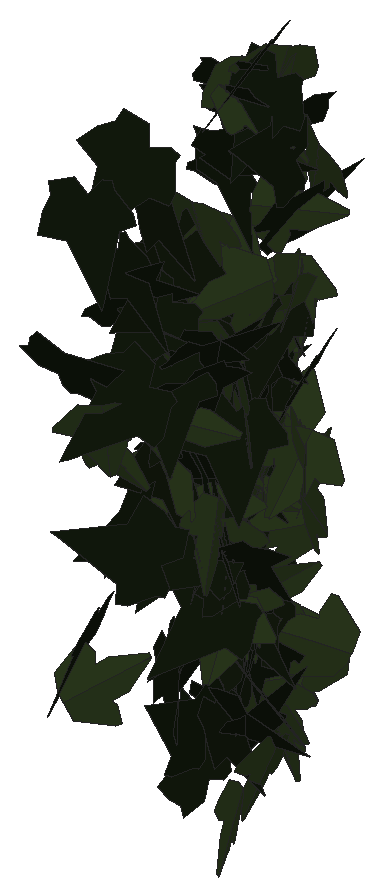
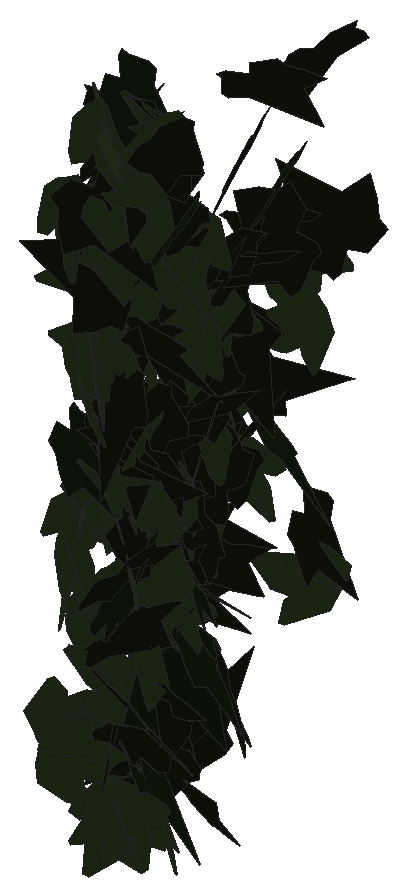
# SketchUp Ruby script. Lengths in inches.
U = 1.inch
M = Sketchup.active_model
def pt(a) = Geom::Point3d.new(a.map { |v| v * U })
def face(e, loops, mat)
  f = e.add_face(loops[0].map { |a| pt(a) })
  loops[1..].each { |l| e.add_face(l.map { |a| pt(a) }).erase! }
  f.material = f.back_material = mat if mat
  f
end
# faces: each face lists its corners as indices into pts; further lists are holes
def faces(e, pts, list, mat = nil) = list.each { |f| face(e, (f[0].is_a?(Array) ? f : [f]).map { |l| l.map { |i| pts[i] } }, mat) }
# xy, xz, yz: faces in a plane at the given z, y or x. An outline is a flat list of corners, or four numbers for a rectangle; further outlines are holes
def ring(l) = l.size == 4 ? [[l[0], l[1]], [l[2], l[1]], [l[2], l[3]], [l[0], l[3]]] : l.each_slice(2).to_a
def flat(e, list, mat, &to3) = list.each { |f| face(e, (f[0].is_a?(Array) ? f : [f]).map { |l| ring(l).map { |u, v| to3.(u, v) } }, mat) }
def xy(e, z, list, mat = nil) = flat(e, list, mat) { |x, y| [x, y, z] }
def xz(e, y, list, mat = nil) = flat(e, list, mat) { |x, z| [x, y, z] }
def yz(e, x, list, mat = nil) = flat(e, list, mat) { |y, z| [x, y, z] }
def lines(e, pts, list) = list.each { |a, b| e.add_line(pt(pts[a]), pt(pts[b])) }
# prism: a flat outline (further loops are holes) pulled along v
def prism(e, loops, v, mat = nil)
  f = face(e, loops, mat); d = Geom::Vector3d.new(v.map { |x| x * U })
  f.pushpull(f.normal.samedirection?(d) ? d.length : -d.length)
end
def box(e, o, s, mat = nil) = prism(e, [[o, [o[0] + s[0], o[1], o[2]], [o[0] + s[0], o[1] + s[1], o[2]], [o[0], o[1] + s[1], o[2]]]], [0, 0, s[2]], mat)
def at(x, y, z, deg = 0) = Geom::Transformation.translation(pt([x, y, z])) * Geom::Transformation.rotation(ORIGIN, Z_AXIS, deg.degrees)
def axes(o, x, y, z) = Geom::Transformation.new([*x, 0, *y, 0, *z, 0, *pt(o).to_a, 1])
def part(name) = M.definitions.add(name)
# library, detail: a bought-in or finely detailed component or shape, given as its bounding box
def library(name, o, s) = part(name).tap { |d| box(d.entities, o, s) }
def detail(e, o, s) = box(e.add_group.entities, o, s)
def put(e, d, t, mat = nil) = e.add_instance(d, t).tap { |i| i.material = mat if mat }
def group(e, t, mat = nil) = e.add_group.tap { |g| g.transformation = t; g.material = mat if mat }.entities
root = M.entities
M.materials.add("efeu1").color = [18, 25, 13]
M.materials.add("efeu2").color = [43, 57, 29]
c1 = part("ivyleaf_9")
p = [[1.54,2.16,1.25],[1.36,2.04,1.19],[-0.21,0.99,0.68],[-0.71,1.11,0.82],[-0.85,0.86,0.67],[-0.8,0.17,0.21],
  [-0.9,-0.01,0.1],[-0.67,-0.16,-0.02],[-0.08,-0.08,-0.05],[-0.03,-0.6,-0.4],[0.65,-0.88,-0.66],[0.83,-0.6,-0.49],
  [1.29,-0.42,-0.43],[1.8125,-0.07,-0.26],[1.21,0.44,0.15]]
faces(c1.entities,p,[[0,1,2,3,4,5,6,7,8,9,10,11,12,13,14]],"efeu1")
c2 = part("ivyleaf_10")
p = [[0,0.5,-0.03],[-0.0625,2.02,-0.43],[-0.19,2.01,-0.46],[-0.54,1.05,-0.29],[-0.52,0.625,-0.18],[-0.83,0.76,-0.28],
  [-1.16,0.64,-0.33],[-1.15,0.33,-0.24],[-0.77,-0.39,0.02],[-0.3,-0.51,0.16],[0.04,-0.48,0.23],[-0.02,2.01,-0.4375],
  [-0.06,2.01,-0.43],[0.04,-0.49,0.23],[0.67,-0.49,0.14],[1.38,0.36,-0.2],[1.375,0.51,-0.24],[0.81,0.65,-0.19],
  [0.62,0.59,-0.15],[0.6,1.09,-0.28],[0.5,1.23,-0.31]]
faces(c2.entities,p,[[0,1,2,3,4,5,6,7,8,9,10],[11,12,0,13,14,15,16,17,18,19,20]],"efeu2")
put(root,c1,axes([52.49,219.07,230.18],[0.03355,-0.19875,0.45757],[0.42754,-0.22487,-0.12902],[0.25707,0.39992,0.15486]))
put(root,c2,axes([53.3,218.97,229.84],[-0.39077,-0.31074,-0.02717],[0.0214,0.01674,-0.49926],[0.31119,-0.39136,0.00022]))
put(root,c1,axes([53.72,219.3,230.26],[-0.45004,-0.19221,0.10255],[-0.09066,-0.04877,-0.48929],[0.19809,-0.459,0.00905]))
put(root,c1,axes([54.02,219.17,227.8],[-0.2114,0.01977,0.45268],[-0.45185,0.02806,-0.21224],[-0.03379,-0.49882,0.006]))
put(root,c1,axes([52.84,219.21,232.84],[0.00085,-0.48604,-0.11732],[0.00176,0.11732,-0.48604],[0.5,0.00041,0.00191]))
put(root,c1,axes([52.77,219.44,226.41],[-0.27604,0.24164,-0.33972],[0.2451,-0.23552,-0.36668],[-0.33723,-0.36897,0.01157]))
put(root,c2,axes([52.78,219.42,229.24],[-0.31286,0.0658,-0.38444],[0.37768,-0.07193,-0.31967],[-0.09737,-0.4904,-0.0047]))
put(root,c2,axes([52.71,219.21,225.41],[0.17923,0.11616,-0.45209],[0.38711,0.2336,0.21349],[0.26082,-0.42654,-0.00619]))
put(root,c1,axes([53.09,219.83,227.77],[-0.36743,0.3333,0.06248],[-0.04862,0.03939,-0.49607],[-0.3356,-0.37062,0.00346]))
put(root,c1,axes([52.82,220.43,233.02],[-0.41171,-0.28303,0.01984],[-0.01039,-0.01989,-0.4995],[0.28353,-0.4117,0.0105]))
put(root,c1,axes([52.59,220.2,231.49],[0.30591,-0.37984,-0.11018],[-0.06702,0.08749,-0.4877],[0.38978,0.31315,0.00262]))
put(root,c1,axes([53.1875,220.51,229.81],[-0.26806,-0.30832,-0.28824],[0.31945,0.07496,-0.37727],[0.27585,-0.38642,0.1568]))
put(root,c1,axes([52.45,220.15,230.8125],[0.28224,0.27787,0.30517],[0.2129,0.2187,-0.39603],[-0.35357,0.3535,0.00513]))
put(root,c1,axes([52.83,220.91,230.51],[-0.32883,-0.35018,0.13873],[-0.03254,-0.15706,-0.47357],[0.37525,-0.32047,0.0805]))
put(root,c1,axes([52.66,221.16,230.56],[-0.08705,-0.25552,0.42087],[-0.14402,-0.39549,-0.26989],[0.47083,-0.16821,-0.00474]))
put(root,c1,axes([53.45,220.52,229.71],[0.17913,0.46548,-0.03522],[-0.01706,-0.03117,-0.49874],[-0.4665,0.17988,0.00472]))
put(root,c1,axes([52.68,221.19,227.96],[0.20703,-0.32676,-0.31681],[0.16838,-0.26836,0.38682],[-0.42283,-0.26686,-0.00108]))
put(root,c1,axes([52.67,220.71,232.24],[0.30016,-0.29801,-0.26663],[-0.20004,0.17676,-0.42277],[0.34624,0.36048,-0.01311]))
put(root,c1,axes([52.84,220.81,229.63],[-0.10996,0.41296,-0.25955],[0.08139,-0.2468,-0.42716],[-0.48092,-0.13619,-0.01294]))
put(root,c2,axes([52.76,220.88,227.96],[0.46781,0.01762,-0.17561],[-0.17545,-0.00761,-0.46814],[-0.01917,0.49963,-0.00094]))
put(root,c2,axes([52.88,220.75,228.93],[-0.08972,-0.1035,-0.48087],[0.465,0.14154,-0.11723],[0.16039,-0.46825,0.07085]))
put(root,c2,axes([52.83,220.77,228.74],[-0.28235,0.34296,0.22947],[-0.20138,0.12817,-0.43934],[-0.36018,-0.34051,0.06575]))
put(root,c1,axes([53.14,220.8,230.125],[0.39895,0.2774,-0.11783],[-0.10096,-0.06117,-0.48586],[-0.28398,0.41147,0.00721]))
put(root,c1,axes([53.07,221.33,223.92],[0.0538,0.0666,0.49262],[-0.30402,-0.38762,0.0856],[0.39329,-0.30874,-0.00121]))
put(root,c2,axes([53.27,221.29,227.3],[-0.0076,-0.39344,0.30846],[0.25408,-0.26872,-0.3365],[0.43056,0.15163,0.20401]))
put(root,c1,axes([53.22,220.84,229.74],[0.22782,0.41878,-0.15074],[0.07738,0.12949,0.4767],[0.4383,-0.24053,-0.0058]))
put(root,c1,axes([53.31,221.375,226.94],[-0.37477,-0.22935,0.23863],[-0.19792,-0.13363,-0.43928],[0.26527,-0.42372,0.00937]))
put(root,c2,axes([53,221.125,229.96],[-0.29644,-0.40088,-0.03766],[0.02235,0.03031,-0.49858],[0.40203,-0.29728,-0.00005]))
put(root,c1,axes([53.45,221.42,226.04],[-0.44352,-0.21328,0.08834],[-0.06435,-0.06954,-0.49094],[0.2217,-0.44685,0.03424]))
put(root,c1,axes([52.38,221.44,225],[-0.09397,-0.09787,-0.48124],[0.48962,-0.05653,-0.08411],[-0.03795,-0.48706,0.10646]))
put(root,c1,axes([53.53,221.45,228.85],[-0.18917,-0.42017,-0.1941],[0.09892,0.16814,-0.46037],[0.45214,-0.21257,0.01951]))
put(root,c2,axes([52.98,221.19,227.33],[-0.28161,0.39206,0.13033],[-0.10652,0.08349,-0.48133],[-0.39918,-0.29886,0.0365]))
put(root,c2,axes([53.5,221.4375,223.01],[0.36667,-0.33589,0.05228],[0.03981,-0.03394,-0.49726],[0.33759,0.36882,0.00185]))
put(root,c1,axes([52.67,221.72,226.85],[-0.34135,-0.35814,0.07223],[-0.04073,-0.06093,-0.4946],[0.36308,-0.34354,0.01242]))
put(root,c2,axes([53.34,221.51,225.82],[0.3701,0.31447,-0.11889],[-0.0902,-0.07746,-0.48566],[-0.32387,0.38093,-0.00061]))
put(root,c1,axes([52.39,221.58,227.88],[0.24936,-0.18678,0.39107],[0.34078,-0.19424,-0.31006],[0.26774,0.42117,0.03043]))
put(root,c2,axes([52.79,221.48,228.5625],[-0.37959,-0.00625,-0.32538],[0.3252,-0.02672,-0.37886],[-0.01265,-0.49925,0.02435]))
put(root,c1,axes([52.65,221.88,228.89],[-0.23497,-0.41311,0.15533],[-0.05823,-0.14542,-0.47483],[0.43749,-0.24123,0.02023]))
put(root,c1,axes([52.55,221.21,228.28],[0.35344,0.28126,0.21442],[0.16578,0.13603,-0.45168],[-0.31241,0.39037,0.00291]))
put(root,c1,axes([53.51,221.55,226.48],[-0.36745,0.23855,0.24099],[-0.27105,0.00691,-0.4201],[-0.20376,-0.43937,0.12424]))
put(root,c1,axes([52.9,221.54,225.53],[-0.37611,0.31934,-0.08101],[0.06176,-0.05242,-0.49339],[-0.32361,-0.38115,-0.00001]))
put(root,c2,axes([53.43,221.29,226.72],[0.17474,-0.17726,-0.43364],[-0.17042,0.40706,-0.23507],[0.43638,0.22995,0.08185]))
put(root,c2,axes([53.2,221.47,226.95],[-0.43674,-0.16708,-0.17704],[0.16293,0.06954,-0.46757],[0.18087,-0.4661,-0.0063]))
put(root,c1,axes([53.4375,221.28,226.74],[0.39564,0.30092,0.05398],[0.03834,0.03875,-0.49702],[-0.30331,0.39742,0.00758]))
put(root,c1,axes([52.82,221.74,226.82],[-0.30962,0.10542,-0.37818],[0.35672,-0.12561,-0.32707],[-0.16397,-0.47234,0.00257]))
put(root,c1,axes([52.56,221.45,231.2],[0.06409,-0.31044,-0.38668],[-0.02515,0.38736,-0.31515],[0.49524,0.05984,0.03403]))
put(root,c1,axes([53.04,221.61,225.47],[-0.20157,0.38935,-0.24037],[0.11296,-0.21218,-0.43843],[-0.44341,-0.23105,-0.00242]))
put(root,c1,axes([52.64,221.375,229.06],[0.14736,0.47242,-0.07146],[0.00901,0.07202,0.4947],[0.47771,-0.14709,0.01272]))
put(root,c2,axes([53.38,221.76,229.02],[-0.20143,0.31743,-0.32964],[0.16757,-0.28399,-0.37586],[-0.42585,-0.26189,0.00802]))
put(root,c2,axes([53.02,221.53,227.32],[0.32969,0.34979,0.13766],[0.08398,0.10994,-0.48048],[-0.3664,0.33994,0.01375]))
put(root,c1,axes([53.06,221.42,223.3],[-0.44212,0.06125,-0.22534],[-0.2223,0.03735,0.44631],[0.0715,0.49483,-0.00579]))
put(root,c1,axes([53.15,221.53,224.3],[0.30001,-0.29259,-0.27274],[-0.19939,0.18617,-0.41903],[0.34676,0.36019,-0.00497]))
put(root,c2,axes([53.375,221.99,230.5],[-0.09498,-0.04392,0.48893],[-0.11205,-0.48291,-0.06515],[0.47794,-0.12194,0.08189]))
put(root,c2,axes([52.74,221.6,229.92],[-0.47538,0.15456,-0.01135],[0.0127,0.00236,-0.49983],[-0.15445,-0.47551,-0.00617]))
put(root,c1,axes([52.63,222.01,227.76],[-0.113,0.02946,0.48617],[-0.05261,-0.4969,0.01788],[0.48421,-0.04711,0.1154]))
put(root,c1,axes([52.51,221.82,227.58],[-0.05056,-0.04488,-0.49541],[0.48962,0.08342,-0.05753],[0.08782,-0.49094,0.03551]))
put(root,c1,axes([53.24,221.55,226.83],[0.31642,-0.12366,-0.36686],[-0.34405,0.12741,-0.3397],[0.1775,0.46741,-0.00446]))
put(root,c2,axes([52.72,221.6875,231.47],[-0.49779,0.04509,-0.01328],[0.01314,-0.00217,-0.49982],[-0.04513,-0.49796,0.00097]))
put(root,c1,axes([52.9,221.71,224.125],[0.39586,-0.08577,0.29315],[0.28892,-0.05052,-0.40493],[0.09909,0.48999,0.00956]))
put(root,c2,axes([53.16,221.8,225.91],[0.43321,0.17902,0.17402],[0.12757,0.14085,-0.46248],[-0.21461,0.4451,0.07636]))
put(root,c2,axes([52.74,221.99,227.93],[-0.12885,0.03423,-0.4819],[0.43323,-0.21253,-0.13093],[-0.2138,-0.45129,0.02511]))
put(root,c2,axes([53.61,222.08,223.57],[0.06572,-0.46319,0.17645],[0.01064,-0.17664,-0.46764],[0.49555,0.06522,-0.01336]))
put(root,c2,axes([52.83,222.08,231.05],[0.23223,0.35628,-0.26294],[-0.1677,-0.20402,-0.42456],[-0.40981,0.28538,0.02473]))
put(root,c1,axes([52.99,221.97,225.69],[0.32967,-0.36468,-0.09125],[0.01884,0.13724,-0.48043],[0.37545,0.31332,0.10423]))
put(root,c1,axes([53.2,221.89,223.69],[0.16403,0.47141,0.02947],[-0.03426,-0.01924,0.49845],[0.47109,-0.16554,0.02599]))
put(root,c1,axes([53.01,222.27,226.12],[-0.11735,-0.00651,-0.48599],[0.47184,-0.12147,-0.11231],[-0.1166,-0.48498,0.03466]))
put(root,c1,axes([53.65,222.5,232.3],[-0.11399,-0.04,0.48519],[-0.19551,-0.4526,-0.08325],[0.44585,-0.2087,0.08755]))
put(root,c1,axes([53.4,221.82,224.85],[-0.02996,0.16513,0.47099],[-0.04741,0.46876,-0.16737],[-0.49684,-0.05469,-0.01243]))
put(root,c1,axes([53.02,222.375,225.2],[-0.45466,-0.16251,-0.12989],[0.12648,0.03192,-0.48268],[0.16517,-0.47178,0.01208]))
put(root,c1,axes([53.12,222.375,230.18],[-0.49732,-0.02831,0.04327],[-0.04277,-0.00993,-0.49807],[0.02906,-0.4991,0.00745]))
put(root,c1,axes([52.94,222.17,224.67],[0.45723,-0.20226,-0.00596],[-0.00443,0.00473,-0.49996],[0.2023,0.45724,0.00253]))
put(root,c2,axes([52.81,222.26,232.99],[0.19101,-0.45809,0.06061],[0.43841,0.15894,-0.18037],[0.14599,0.12205,0.46238]))
put(root,c1,axes([53.21,222.57,230.05],[-0.13851,-0.47968,-0.02687],[0.00764,0.02576,-0.49928],[0.48037,-0.13872,0.0002]))
put(root,c1,axes([53.34,222.49,233.35],[-0.45384,-0.1327,-0.16255],[0.15238,0.05788,-0.47268],[0.14426,-0.47858,-0.01209]))
put(root,c1,axes([52.75,222.02,228.5],[0.04855,0.05198,0.49491],[0.41248,0.27398,-0.06924],[-0.27839,0.41501,-0.01628]))
put(root,c1,axes([52.59,222.09,232.16],[0.35246,0.14936,0.32165],[0.30226,0.11067,-0.38261],[-0.18549,0.46416,-0.01228]))
put(root,c1,axes([53.03,222.32,224.2],[-0.34643,0.3605,0.00506],[-0.00383,0.00333,-0.49997],[-0.36052,-0.34645,0.00046]))
put(root,c1,axes([53.15,222.55,233.75],[-0.31421,0.26485,-0.28483],[0.1516,-0.2538,-0.40324],[-0.35818,-0.33976,0.07918]))
put(root,c1,axes([53.33,222.18,225.14],[0.13643,-0.08719,-0.47306],[-0.39105,0.26624,-0.16185],[0.28012,0.41414,0.00445]))
put(root,c2,axes([52.76,222.41,229],[-0.09638,0.48756,-0.05471],[0.00718,-0.05434,-0.49699],[-0.49057,-0.09659,0.00347]))
put(root,c1,axes([52.36,222.65,231.83],[0.19337,-0.4442,0.12366],[0.06499,-0.1065,-0.48418],[0.45649,0.20332,0.01656]))
put(root,c2,axes([52.73,222.55,233.18],[0.24429,0.42964,-0.07569],[-0.0334,-0.06807,-0.49422],[-0.43498,0.24652,-0.00456]))
put(root,c1,axes([52.68,222.36,232.93],[0.47348,0.13704,-0.08386],[-0.07924,-0.02783,-0.4929],[-0.13976,0.48005,-0.00464]))
put(root,c1,axes([52.77,222.7,224.56],[0.4812,-0.06201,0.12084],[-0.11929,0.01972,0.48516],[-0.06493,-0.49575,0.00419]))
put(root,c2,axes([53.49,222.93,229.82],[-0.05918,-0.09513,-0.48729],[-0.17198,-0.45643,0.10999],[-0.46575,0.18062,0.02131]))
put(root,c1,axes([52.68,222.59,227.42],[0.12175,0.40068,0.27318],[-0.10005,-0.25485,0.41838],[0.47452,-0.15654,0.01812]))
put(root,c2,axes([53.14,222.67,227.87],[0.06617,-0.4936,0.0445],[0.00086,-0.04478,-0.49799],[0.4956,0.06598,-0.00508]))
put(root,c2,axes([53.64,222.72,227.84],[0.28288,0.3383,-0.23566],[-0.16199,-0.17161,-0.44081],[-0.37913,0.32574,0.01251]))
put(root,c1,axes([52.92,222.2,225.16],[0.02098,0.19858,0.4584],[0.02067,0.45806,-0.19938],[-0.49913,0.02731,0.01101]))
put(root,c1,axes([52.96,222.45,229.29],[0.32936,0.24132,-0.28859],[-0.2558,-0.13759,-0.40698],[-0.27584,0.41574,0.03283]))
put(root,c1,axes([52.62,222.7,228.81],[-0.19137,-0.10789,-0.44915],[0.41917,0.16374,-0.21792],[0.19411,-0.45995,0.02778]))
put(root,c2,axes([52.55,222.5,227.14],[-0.19375,-0.06346,-0.45654],[0.44339,0.10967,-0.20341],[0.12596,-0.48368,0.01378]))
put(root,c2,axes([53.25,223.02,230.0625],[0.04849,-0.12817,0.48086],[0.11899,-0.46613,-0.13624],[0.48321,0.12764,-0.0147]))
put(root,c1,axes([52.62,222.51,233.24],[0.38065,0.2691,-0.1808],[-0.15181,-0.09844,-0.46612],[-0.28646,0.40975,0.00676]))
put(root,c2,axes([53.32,223.07,226.45],[-0.04857,0.07748,0.49157],[-0.07838,-0.48893,0.06932],[0.49142,-0.07033,0.05964]))
put(root,c1,axes([53.03,222.64,228.26],[-0.13297,0.14589,0.45939],[-0.40555,0.22367,-0.18842],[-0.26047,-0.42272,0.05885]))
put(root,c2,axes([52.96,222.93,232.83],[0.22705,-0.35771,-0.2655],[0.19021,-0.19162,0.42084],[-0.40283,-0.2921,0.04906]))
put(root,c2,axes([52.55,222.67,228.0625],[0.22728,0.13135,0.42555],[0.361,0.22544,-0.26239],[-0.26081,0.42652,0.00764]))
put(root,c2,axes([53.13,222.76,223.7],[-0.45247,0.19641,-0.08184],[0.07405,-0.03492,-0.49325],[-0.19948,-0.45848,0.00251]))
put(root,c2,axes([52.86,222.7,225.33],[-0.19043,-0.26383,0.37964],[0.26893,0.27075,0.32306],[-0.37605,0.32724,0.03879]))
put(root,c1,axes([53.13,222.88,225.38],[-0.45776,0.18089,0.08796],[-0.08472,0.02491,-0.49214],[-0.18243,-0.46546,0.00784]))
put(root,c2,axes([53.12,222.95,233.41],[-0.2499,-0.42007,0.10533],[-0.05295,-0.09106,-0.48878],[0.42982,-0.25544,0.00102]))
put(root,c2,axes([53.81,223.1,224.76],[0.11641,0.15718,0.46016],[-0.26115,-0.37892,0.19549],[0.41018,-0.28585,-0.00612]))
put(root,c2,axes([52.69,222.96,232.45],[-0.17629,0.09105,-0.45895],[0.42237,-0.18004,-0.19796],[-0.2013,-0.45749,-0.01343]))
put(root,c2,axes([53.33,223.05,229.49],[0.35489,-0.32892,0.12597],[0.09936,-0.07806,-0.48377],[0.33791,0.3684,0.00996]))
put(root,c2,axes([52.92,222.83,223.82],[-0.42085,-0.19336,-0.1884],[0.16936,0.08264,-0.46313],[0.21024,-0.45363,-0.00407]))
put(root,c2,axes([53.29,223.01,228.02],[0.19444,0.17717,0.42521],[-0.37738,-0.20341,0.25732],[0.26416,-0.421,0.05462]))
put(root,c2,axes([53.7,222.59,227.78],[0.05866,0.035,-0.49531],[-0.17529,0.4681,0.01231],[0.46458,0.17221,0.06719]))
put(root,c2,axes([53.23,222.95,230.2],[0.47095,0.11209,0.12506],[0.12036,0.03436,-0.48408],[-0.11711,0.48606,0.00538]))
put(root,c2,axes([53.08,222.73,231.3],[-0.05485,-0.09121,-0.48854],[0.42937,0.23881,-0.09279],[0.25026,-0.42971,0.05213]))
put(root,c2,axes([52.98,222.7,227.34],[-0.03489,0.14591,0.47696],[-0.41371,0.25861,-0.10938],[-0.27862,-0.40228,0.10268]))
put(root,c1,axes([52.66,223.24,227.33],[-0.07525,-0.49221,0.04551],[-0.0025,-0.04565,-0.49791],[0.4943,-0.07516,0.00441]))
put(root,c2,axes([53.75,222.7,227.07],[-0.20187,0.31964,0.32724],[-0.19894,0.26074,-0.37741],[-0.41191,-0.28258,0.02191]))
put(root,c2,axes([53.32,222.95,230.16],[0.2374,-0.41006,-0.15967],[-0.06533,0.14658,-0.47355],[0.43517,0.2457,0.01602]))
put(root,c1,axes([53.1875,222.68,231.02],[0.06925,0.45885,-0.18617],[-0.03959,0.19251,0.45975],[0.4936,-0.04894,0.063]))
put(root,c1,axes([52.62,223.35,226.55],[-0.19214,-0.43222,0.16208],[-0.06289,-0.14941,-0.47299],[0.4573,-0.20215,0.00305]))
put(root,c1,axes([52.89,222.875,229.75],[0.38605,0.01021,-0.31759],[-0.31723,-0.0161,-0.38614],[-0.01811,0.49964,-0.00595]))
put(root,c1,axes([53.51,223.1,228.92],[-0.29939,0.31193,-0.25113],[0.16669,-0.18803,-0.43227],[-0.36412,-0.34256,0.0086]))
put(root,c2,axes([52.77,223.36,231.9],[-0.21515,-0.23195,-0.38718],[-0.16455,-0.35909,0.30656],[-0.42028,0.25933,0.07818]))
put(root,c2,axes([52.42,223,232.47],[-0.20613,0.00252,-0.45553],[0.45549,-0.00589,-0.20615],[-0.0064,-0.49996,0.00013]))
put(root,c2,axes([53.55,223.32,224.49],[-0.07834,-0.03828,0.49234],[-0.29237,-0.39814,-0.07748],[0.39797,-0.30003,0.03999]))
put(root,c1,axes([52.8,223.28,226.68],[0.23095,-0.43479,0.08731],[-0.03356,0.08102,0.49225],[-0.4422,-0.23323,0.00824]))
put(root,c2,axes([52.72,223.17,223.91],[0.32405,0.3535,-0.14152],[-0.09753,-0.10257,-0.47955],[-0.36807,0.3384,0.00248]))
put(root,c2,axes([53.68,223.04,232.15],[-0.41511,0.11273,0.2549],[-0.24567,0.06797,-0.43014],[-0.13164,-0.48236,-0.00104]))
put(root,c1,axes([53.07,223.2,232.52],[-0.12325,0.38796,-0.29034],[-0.01827,-0.30309,-0.39724],[-0.48423,-0.08731,0.08889]))
put(root,c2,axes([53.38,223.32,227.49],[0.10886,-0.47318,0.11936],[0.04146,-0.11288,-0.48532],[0.48624,0.11557,0.01466]))
